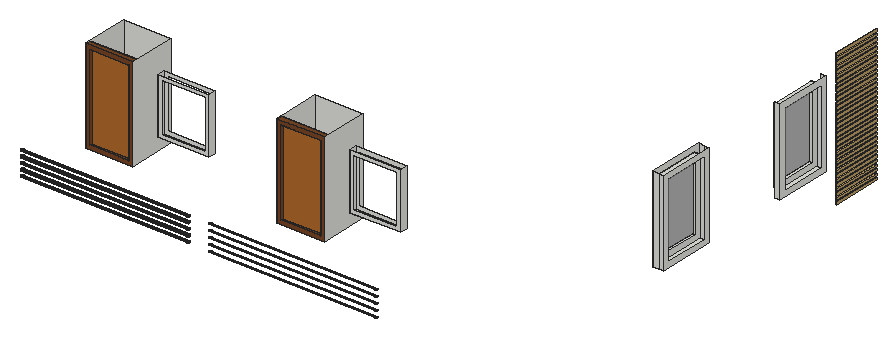
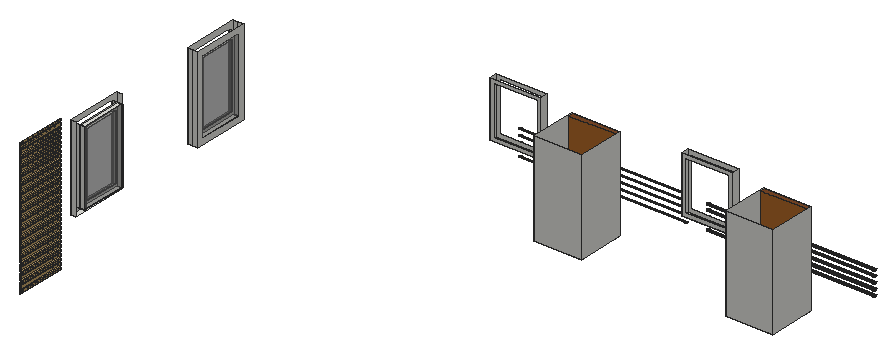
# SketchUp Ruby script. Lengths in inches.
U = 1.inch
M = Sketchup.active_model
def pt(a) = Geom::Point3d.new(a.map { |v| v * U })
def face(e, loops, mat)
  f = e.add_face(loops[0].map { |a| pt(a) })
  loops[1..].each { |l| e.add_face(l.map { |a| pt(a) }).erase! }
  f.material = f.back_material = mat if mat
  f
end
# faces: each face lists its corners as indices into pts; further lists are holes
def faces(e, pts, list, mat = nil) = list.each { |f| face(e, (f[0].is_a?(Array) ? f : [f]).map { |l| l.map { |i| pts[i] } }, mat) }
# xy, xz, yz: faces in a plane at the given z, y or x. An outline is a flat list of corners, or four numbers for a rectangle; further outlines are holes
def ring(l) = l.size == 4 ? [[l[0], l[1]], [l[2], l[1]], [l[2], l[3]], [l[0], l[3]]] : l.each_slice(2).to_a
def flat(e, list, mat, &to3) = list.each { |f| face(e, (f[0].is_a?(Array) ? f : [f]).map { |l| ring(l).map { |u, v| to3.(u, v) } }, mat) }
def xy(e, z, list, mat = nil) = flat(e, list, mat) { |x, y| [x, y, z] }
def xz(e, y, list, mat = nil) = flat(e, list, mat) { |x, z| [x, y, z] }
def yz(e, x, list, mat = nil) = flat(e, list, mat) { |y, z| [x, y, z] }
def lines(e, pts, list) = list.each { |a, b| e.add_line(pt(pts[a]), pt(pts[b])) }
# prism: a flat outline (further loops are holes) pulled along v
def prism(e, loops, v, mat = nil)
  f = face(e, loops, mat); d = Geom::Vector3d.new(v.map { |x| x * U })
  f.pushpull(f.normal.samedirection?(d) ? d.length : -d.length)
end
def box(e, o, s, mat = nil) = prism(e, [[o, [o[0] + s[0], o[1], o[2]], [o[0] + s[0], o[1] + s[1], o[2]], [o[0], o[1] + s[1], o[2]]]], [0, 0, s[2]], mat)
def at(x, y, z, deg = 0) = Geom::Transformation.translation(pt([x, y, z])) * Geom::Transformation.rotation(ORIGIN, Z_AXIS, deg.degrees)
def axes(o, x, y, z) = Geom::Transformation.new([*x, 0, *y, 0, *z, 0, *pt(o).to_a, 1])
def part(name) = M.definitions.add(name)
# library, detail: a bought-in or finely detailed component or shape, given as its bounding box
def library(name, o, s) = part(name).tap { |d| box(d.entities, o, s) }
def detail(e, o, s) = box(e.add_group.entities, o, s)
def put(e, d, t, mat = nil) = e.add_instance(d, t).tap { |i| i.material = mat if mat }
def group(e, t, mat = nil) = e.add_group.tap { |g| g.transformation = t; g.material = mat if mat }.entities
root = M.entities
M.materials.add("Generic").color = [191, 159, 103]
M.materials.add("[Translucent Glass Gray]").color = [128, 128, 128]
M.materials["[Translucent Glass Gray]"].alpha = 0.5
M.materials.add("[Wood Bamboo]").color = [177, 105, 43]
M.materials.add("[Wood Veneer 01]").color = [120, 70, 37]
c1 = part("Group\#5")
xy(c1.entities,0,[[0,0,1,57.75]])
xy(c1.entities,2.57,[[0,0,1,57.75]])
xz(c1.entities,0,[[0,0,1,2.57]])
xz(c1.entities,57.75,[[0,0,1,2.57]])
yz(c1.entities,1,[[0,0,57.75,2.57]])
c2 = part("Group\#6")
put(c2.entities,c1,at(0,0,4.75))
put(c2.entities,c1,at(0,0,0))
put(c2.entities,c1,at(0,0,19))
put(c2.entities,c1,at(0,0,28.5))
put(c2.entities,c1,at(0,0,133))
put(c2.entities,c1,at(0,0,152))
put(c2.entities,c1,at(0,0,128.25))
put(c2.entities,c1,at(0,0,9.5))
put(c2.entities,c1,at(0,0,123.5))
put(c2.entities,c1,at(0,0,114))
put(c2.entities,c1,at(0,0,147.25))
put(c2.entities,c1,at(0,0,118.75))
put(c2.entities,c1,at(0,0,142.5))
put(c2.entities,c1,at(0,0,109.25))
put(c2.entities,c1,at(0,0,137.75))
put(c2.entities,c1,at(0,0,104.5))
put(c2.entities,c1,at(0,0,99.75))
put(c2.entities,c1,at(0,0,95))
put(c2.entities,c1,at(0,0,85.5))
put(c2.entities,c1,at(0,0,80.75))
put(c2.entities,c1,at(0,0,90.25))
put(c2.entities,c1,at(0,0,76))
put(c2.entities,c1,at(0,0,71.25))
put(c2.entities,c1,at(0,0,38))
put(c2.entities,c1,at(0,0,14.25))
put(c2.entities,c1,at(0,0,33.25))
put(c2.entities,c1,at(0,0,57))
put(c2.entities,c1,at(0,0,23.75))
put(c2.entities,c1,at(0,0,61.75))
put(c2.entities,c1,at(0,0,156.75))
put(c2.entities,c1,at(0,0,47.5))
put(c2.entities,c1,at(0,0,52.25))
put(c2.entities,c1,at(0,0,42.75))
put(c2.entities,c1,at(0,0,66.5))
c3 = part("Group\#4")
xy(c3.entities,0,[[0,0,55.6875,6]],"[Wood Veneer 01]")
xy(c3.entities,4.75,[[4.75,0,50.9375,3]],"[Wood Veneer 01]")
xy(c3.entities,105.5,[[4.75,0,50.9375,3]],"[Wood Veneer 01]")
xy(c3.entities,110.25,[[0,0,55.6875,6]],"[Wood Veneer 01]")
xz(c3.entities,0,[[[0,0,55.6875,110.25],[4.75,4.75,50.9375,105.5]]],"[Wood Veneer 01]")
xz(c3.entities,3,[[4.75,4.75,50.9375,105.5]],"[Wood Bamboo]")
xz(c3.entities,6,[[0,0,55.6875,110.25]],"[Wood Bamboo]")
yz(c3.entities,0,[[0,0,6,110.25]],"[Wood Veneer 01]")
yz(c3.entities,4.75,[[0,4.75,3,105.5]],"[Wood Veneer 01]")
yz(c3.entities,50.9375,[[0,4.75,3,105.5]],"[Wood Veneer 01]")
yz(c3.entities,55.6875,[[0,0,6,110.25]],"[Wood Veneer 01]")
c4 = part("Group\#7")
xy(c4.entities,0,[[0,0,6,54.3125]])
xy(c4.entities,5.9,[[3,5.9,6,48.41]])
xy(c4.entities,81.98,[[3,5.9,6,48.41]])
xy(c4.entities,87.88,[[0,0,6,54.3125]])
xz(c4.entities,0,[[0,0,6,87.88]])
xz(c4.entities,5.9,[[3,5.9,6,81.98]])
xz(c4.entities,48.41,[[3,5.9,6,81.98]])
xz(c4.entities,54.3125,[[0,0,6,87.88]])
yz(c4.entities,0,[[0,0,54.3125,87.88]],"[Translucent Glass Gray]")
yz(c4.entities,3,[[5.9,5.9,48.41,81.98]],"[Translucent Glass Gray]")
yz(c4.entities,6,[[[0,0,54.3125,87.88],[5.9,5.9,48.41,81.98]]])
xy(root,234.72,[[214.375,158.75,270.0625,214.75],[439.6875,158.75,495.375,214.75]])
xy(root,272.84,[[802.875,257.24,809.375,324.36],[809.375,257.24,815.3125,324.36],[809.375,428.47,815.3125,495.59]])
xy(root,279.25,[[802.875,263.64,815.3125,317.96],[802.875,434.88,815.3125,489.19]])
xy(root,282.21,[[306.72,150.125,366.62,158.75],[532.04,150.125,591.93,158.75]])
xz(root,150.125,[[[306.72,282.21,366.62,348.04],[310.76,286.25,362.58,344]],[[532.04,282.21,591.93,348.04],[536.08,286.25,587.89,344]]])
xz(root,158.75,[[[306.72,282.21,366.62,348.04],[310.76,286.25,362.58,344]],[[532.04,282.21,591.93,348.04],[536.08,286.25,587.89,344]]])
xz(root,214.75,[[214.375,234.72,270.0625,344.97],[439.6875,234.72,495.375,344.97]])
xz(root,257.24,[[802.875,272.84,809.375,373.53],[809.375,272.84,815.3125,373.53]])
xz(root,263.64,[[802.875,279.25,815.3125,367.13]])
xz(root,317.96,[[802.875,279.25,815.3125,367.13]])
xz(root,324.36,[[802.875,272.84,809.375,373.53],[809.375,272.84,815.3125,373.53]])
xz(root,428.47,[[809.375,272.84,815.3125,373.53]])
xz(root,434.88,[[802.875,279.25,815.3125,367.13]])
xz(root,489.19,[[802.875,279.25,815.3125,367.13]])
xz(root,495.59,[[809.375,272.84,815.3125,373.53]])
yz(root,214.375,[[158.75,234.72,214.75,344.97]])
yz(root,270.0625,[[158.75,234.72,214.75,344.97]])
yz(root,306.72,[[150.125,282.21,158.75,348.04]])
yz(root,366.62,[[150.125,282.21,158.75,348.04]])
yz(root,439.6875,[[158.75,234.72,214.75,344.97]])
yz(root,495.375,[[158.75,234.72,214.75,344.97]])
yz(root,532.04,[[150.125,282.21,158.75,348.04]])
yz(root,591.93,[[150.125,282.21,158.75,348.04]])
yz(root,802.875,[[[257.24,272.84,324.36,373.53],[263.64,279.25,317.96,367.13]]])
yz(root,815.3125,[[[257.24,272.84,324.36,373.53],[263.64,279.25,317.96,367.13]],[[428.47,272.84,495.59,373.53],[434.88,279.25,489.19,367.13]]])
p = [[415.53,88.8125,226.625],[415.53,88.93,226.54],[613.23,88.93,226.54],[613.23,88.8125,226.625],[415.53,89.0625,226.48],[613.23,89.0625,226.48],
  [415.53,89.21,226.46],[613.23,89.21,226.46],[415.53,89.36,226.48],[613.23,89.36,226.48],[415.53,89.49,226.54],[613.23,89.49,226.54],
  [415.53,89.61,226.625],[613.23,89.61,226.625],[415.53,88.72,226.74],[613.23,88.72,226.74],[415.53,89.7,226.74],[613.23,89.7,226.74],
  [415.53,88.67,226.88],[613.23,88.67,226.88],[415.53,89.75,226.88],[613.23,89.75,226.88],[415.53,88.65,227.02],[613.23,88.65,227.02],
  [415.53,89.77,227.02],[613.23,89.77,227.02],[415.53,88.67,227.17],[613.23,88.67,227.17],[415.53,89.75,227.17],[613.23,89.75,227.17],
  [193.83,89.44,227.24],[193.83,89.73,227.125],[391.53,89.73,227.125],[391.53,89.44,227.24],[193.83,90.04,227.08],[391.53,90.04,227.08],
  [193.83,90.35,227.125],[391.53,90.35,227.125],[193.83,90.63,227.24],[391.53,90.63,227.24],[415.53,88.72,227.31],[613.23,88.72,227.31],
  [193.83,89.2,227.43],[391.53,89.2,227.43],[415.53,89.7,227.31],[613.23,89.7,227.31],[193.83,90.88,227.43],[391.53,90.88,227.43],
  [415.53,88.8125,227.42],[613.23,88.8125,227.42],[415.53,89.61,227.42],[613.23,89.61,227.42],[415.53,88.93,227.51],[613.23,88.93,227.51],
  [193.83,89.01,227.68],[391.53,89.01,227.68],[415.53,89.49,227.51],[613.23,89.49,227.51],[193.83,91.07,227.68],[391.53,91.07,227.68],
  [415.53,89.0625,227.57],[613.23,89.0625,227.57],[415.53,89.36,227.57],[613.23,89.36,227.57],[415.53,89.21,227.59],[613.23,89.21,227.59],
  [193.83,88.89,227.96],[391.53,88.89,227.96],[193.83,91.18,227.96],[391.53,91.18,227.96],[193.83,88.85,228.27],[391.53,88.85,228.27],
  [193.83,91.23,228.27],[391.53,91.23,228.27],[193.83,88.89,228.58],[391.53,88.89,228.58],[193.83,91.18,228.58],[391.53,91.18,228.58],
  [193.83,89.01,228.86],[391.53,89.01,228.86],[193.83,91.07,228.86],[391.53,91.07,228.86],[193.83,89.2,229.11],[391.53,89.2,229.11],
  [193.83,90.88,229.11],[391.53,90.88,229.11],[193.83,89.44,229.3],[391.53,89.44,229.3],[193.83,90.63,229.3],[391.53,90.63,229.3],
  [193.83,89.73,229.42],[391.53,89.73,229.42],[193.83,90.35,229.42],[391.53,90.35,229.42],[193.83,90.04,229.46],[391.53,90.04,229.46],
  [415.53,89.0625,233.86],[415.53,89.21,233.84],[613.23,89.21,233.84],[613.23,89.0625,233.86],[415.53,89.36,233.86],[613.23,89.36,233.86],
  [193.83,89.44,233.93],[193.83,89.73,233.8125],[391.53,89.73,233.8125],[391.53,89.44,233.93],[193.83,90.04,233.77],[391.53,90.04,233.77],
  [193.83,90.35,233.8125],[391.53,90.35,233.8125],[193.83,90.63,233.93],[391.53,90.63,233.93],[415.53,88.8125,234],[415.53,88.93,233.91],
  [613.23,88.93,233.91],[613.23,88.8125,234],[193.83,89.2,234.12],[391.53,89.2,234.12],[415.53,89.49,233.91],[613.23,89.49,233.91],
  [415.53,89.61,234],[613.23,89.61,234],[193.83,90.88,234.12],[391.53,90.88,234.12],[415.53,88.72,234.12],[613.23,88.72,234.12],
  [415.53,89.7,234.12],[613.23,89.7,234.12],[415.53,88.67,234.25],[613.23,88.67,234.25],[193.83,89.01,234.36],[391.53,89.01,234.36],
  [415.53,89.75,234.25],[613.23,89.75,234.25],[193.83,91.07,234.36],[391.53,91.07,234.36],[415.53,88.65,234.4],[613.23,88.65,234.4],
  [415.53,89.77,234.4],[613.23,89.77,234.4],[415.53,88.67,234.54],[613.23,88.67,234.54],[193.83,88.89,234.65],[391.53,88.89,234.65],
  [415.53,89.75,234.54],[613.23,89.75,234.54],[193.83,91.18,234.65],[391.53,91.18,234.65],[415.53,88.72,234.68],[613.23,88.72,234.68],
  [415.53,89.7,234.68],[613.23,89.7,234.68],[415.53,88.8125,234.8],[613.23,88.8125,234.8],[193.83,88.85,234.96],[391.53,88.85,234.96],
  [415.53,89.61,234.8],[613.23,89.61,234.8],[193.83,91.23,234.96],[391.53,91.23,234.96],[415.53,88.93,234.89],[613.23,88.93,234.89],
  [415.53,89.49,234.89],[613.23,89.49,234.89],[415.53,89.0625,234.94],[613.23,89.0625,234.94],[415.53,89.21,234.96],[613.23,89.21,234.96],
  [415.53,89.36,234.94],[613.23,89.36,234.94],[193.83,88.89,235.27],[391.53,88.89,235.27],[193.83,91.18,235.27],[391.53,91.18,235.27],
  [193.83,89.01,235.55],[391.53,89.01,235.55],[193.83,91.07,235.55],[391.53,91.07,235.55],[193.83,89.2,235.8],[391.53,89.2,235.8],
  [193.83,90.88,235.8],[391.53,90.88,235.8],[193.83,89.44,235.99],[391.53,89.44,235.99],[193.83,90.63,235.99],[391.53,90.63,235.99],
  [193.83,89.73,236.11],[391.53,89.73,236.11],[193.83,90.35,236.11],[391.53,90.35,236.11],[193.83,90.04,236.15],[391.53,90.04,236.15],
  [193.83,89.44,240.93],[193.83,89.73,240.8125],[391.53,89.73,240.8125],[391.53,89.44,240.93],[193.83,90.04,240.77],[391.53,90.04,240.77],
  [193.83,90.35,240.8125],[391.53,90.35,240.8125],[193.83,90.63,240.93],[391.53,90.63,240.93],[193.83,89.2,241.12],[391.53,89.2,241.12],
  [193.83,90.88,241.12],[391.53,90.88,241.12],[193.83,89.01,241.36],[391.53,89.01,241.36],[193.83,91.07,241.36],[391.53,91.07,241.36],
  [415.53,89.0625,241.36],[415.53,89.21,241.34],[613.23,89.21,241.34],[613.23,89.0625,241.36],[415.53,89.36,241.36],[613.23,89.36,241.36],
  [415.53,88.8125,241.5],[415.53,88.93,241.41],[613.23,88.93,241.41],[613.23,88.8125,241.5],[193.83,88.89,241.65],[391.53,88.89,241.65],
  [415.53,89.49,241.41],[613.23,89.49,241.41],[415.53,89.61,241.5],[613.23,89.61,241.5],[193.83,91.18,241.65],[391.53,91.18,241.65],
  [415.53,88.72,241.62],[613.23,88.72,241.62],[415.53,89.7,241.62],[613.23,89.7,241.62],[415.53,88.67,241.75],[613.23,88.67,241.75],
  [415.53,89.75,241.75],[613.23,89.75,241.75],[193.83,88.85,241.96],[391.53,88.85,241.96],[193.83,91.23,241.96],[391.53,91.23,241.96],
  [415.53,88.65,241.9],[613.23,88.65,241.9],[415.53,89.77,241.9],[613.23,89.77,241.9],[415.53,88.67,242.04],[613.23,88.67,242.04],
  [415.53,89.75,242.04],[613.23,89.75,242.04],[415.53,88.72,242.18],[613.23,88.72,242.18],[193.83,88.89,242.27],[391.53,88.89,242.27],
  [415.53,89.7,242.18],[613.23,89.7,242.18],[193.83,91.18,242.27],[391.53,91.18,242.27],[415.53,88.8125,242.3],[613.23,88.8125,242.3],
  [415.53,89.61,242.3],[613.23,89.61,242.3],[415.53,88.93,242.39],[613.23,88.93,242.39],[193.83,89.01,242.55],[391.53,89.01,242.55],
  [415.53,89.49,242.39],[613.23,89.49,242.39],[193.83,91.07,242.55],[391.53,91.07,242.55],[415.53,89.0625,242.44],[613.23,89.0625,242.44],
  [415.53,89.21,242.46],[613.23,89.21,242.46],[415.53,89.36,242.44],[613.23,89.36,242.44],[193.83,89.2,242.8],[391.53,89.2,242.8],
  [193.83,90.88,242.8],[391.53,90.88,242.8],[193.83,89.44,242.99],[391.53,89.44,242.99],[193.83,90.63,242.99],[391.53,90.63,242.99],
  [193.83,89.73,243.11],[391.53,89.73,243.11],[193.83,90.35,243.11],[391.53,90.35,243.11],[193.83,90.04,243.15],[391.53,90.04,243.15],
  [193.83,89.44,247.93],[193.83,89.73,247.8125],[391.53,89.73,247.8125],[391.53,89.44,247.93],[193.83,90.04,247.77],[391.53,90.04,247.77],
  [193.83,90.35,247.8125],[391.53,90.35,247.8125],[193.83,90.63,247.93],[391.53,90.63,247.93],[193.83,89.2,248.12],[391.53,89.2,248.12],
  [193.83,90.88,248.12],[391.53,90.88,248.12],[193.83,89.01,248.36],[391.53,89.01,248.36],[193.83,91.07,248.36],[391.53,91.07,248.36],
  [193.83,88.89,248.65],[391.53,88.89,248.65],[193.83,91.18,248.65],[391.53,91.18,248.65],[193.83,88.85,248.96],[391.53,88.85,248.96],
  [193.83,91.23,248.96],[391.53,91.23,248.96],[415.53,89.0625,248.86],[415.53,89.21,248.84],[613.23,89.21,248.84],[613.23,89.0625,248.86],
  [415.53,89.36,248.86],[613.23,89.36,248.86],[415.53,88.8125,249],[415.53,88.93,248.91],[613.23,88.93,248.91],[613.23,88.8125,249],
  [415.53,89.49,248.91],[613.23,89.49,248.91],[415.53,89.61,249],[613.23,89.61,249],[415.53,88.72,249.12],[613.23,88.72,249.12],
  [193.83,88.89,249.27],[391.53,88.89,249.27],[415.53,89.7,249.12],[613.23,89.7,249.12],[193.83,91.18,249.27],[391.53,91.18,249.27],
  [415.53,88.67,249.25],[613.23,88.67,249.25],[415.53,89.75,249.25],[613.23,89.75,249.25],[415.53,88.65,249.4],[613.23,88.65,249.4],
  [193.83,89.01,249.55],[391.53,89.01,249.55],[415.53,89.77,249.4],[613.23,89.77,249.4],[193.83,91.07,249.55],[391.53,91.07,249.55],
  [415.53,88.67,249.54],[613.23,88.67,249.54],[415.53,89.75,249.54],[613.23,89.75,249.54],[415.53,88.72,249.68],[613.23,88.72,249.68],
  [415.53,89.7,249.68],[613.23,89.7,249.68],[193.83,89.2,249.8],[391.53,89.2,249.8],[193.83,90.88,249.8],[391.53,90.88,249.8],
  [415.53,88.8125,249.8],[613.23,88.8125,249.8],[415.53,89.61,249.8],[613.23,89.61,249.8],[415.53,88.93,249.89],[613.23,88.93,249.89],
  [193.83,89.44,249.99],[391.53,89.44,249.99],[415.53,89.49,249.89],[613.23,89.49,249.89],[193.83,90.63,249.99],[391.53,90.63,249.99],
  [415.53,89.0625,249.94],[613.23,89.0625,249.94],[415.53,89.21,249.96],[613.23,89.21,249.96],[415.53,89.36,249.94],[613.23,89.36,249.94],
  [193.83,89.73,250.11],[391.53,89.73,250.11],[193.83,90.35,250.11],[391.53,90.35,250.11],[193.83,90.04,250.15],[391.53,90.04,250.15],
  [193.83,89.73,254.375],[193.83,90.04,254.33],[391.53,90.04,254.33],[391.53,89.73,254.375],[193.83,90.35,254.375],[391.53,90.35,254.375],
  [193.83,89.44,254.49],[391.53,89.44,254.49],[193.83,90.63,254.49],[391.53,90.63,254.49],[193.83,89.2,254.68],[391.53,89.2,254.68],
  [193.83,90.88,254.68],[391.53,90.88,254.68],[193.83,89.01,254.93],[391.53,89.01,254.93],[193.83,91.07,254.93],[391.53,91.07,254.93],
  [193.83,88.89,255.21],[391.53,88.89,255.21],[193.83,91.18,255.21],[391.53,91.18,255.21],[193.83,88.85,255.52],[391.53,88.85,255.52],
  [193.83,91.23,255.52],[391.53,91.23,255.52],[193.83,88.89,255.83],[391.53,88.89,255.83],[193.83,91.18,255.83],[391.53,91.18,255.83],
  [193.83,89.01,256.11],[391.53,89.01,256.11],[193.83,91.07,256.11],[391.53,91.07,256.11],[193.83,89.2,256.36],[391.53,89.2,256.36],
  [193.83,90.88,256.36],[391.53,90.88,256.36],[415.53,88.8125,256.4375],[415.53,88.93,256.35],[613.23,88.93,256.35],[613.23,88.8125,256.4375],
  [415.53,89.0625,256.29],[613.23,89.0625,256.29],[415.53,89.21,256.27],[613.23,89.21,256.27],[415.53,89.36,256.29],[613.23,89.36,256.29],
  [415.53,89.49,256.35],[613.23,89.49,256.35],[415.53,89.61,256.4375],[613.23,89.61,256.4375],[415.53,88.72,256.56],[613.23,88.72,256.56],
  [193.83,89.44,256.55],[391.53,89.44,256.55],[415.53,89.7,256.56],[613.23,89.7,256.56],[193.83,90.63,256.55],[391.53,90.63,256.55],
  [193.83,89.73,256.67],[391.53,89.73,256.67],[193.83,90.35,256.67],[391.53,90.35,256.67],[415.53,88.67,256.69],[613.23,88.67,256.69],
  [415.53,89.75,256.69],[613.23,89.75,256.69],[415.53,88.65,256.84],[613.23,88.65,256.84],[193.83,90.04,256.71],[391.53,90.04,256.71],
  [415.53,89.77,256.84],[613.23,89.77,256.84],[415.53,88.67,256.98],[613.23,88.67,256.98],[415.53,89.75,256.98],[613.23,89.75,256.98],
  [415.53,88.72,257.12],[613.23,88.72,257.12],[415.53,89.7,257.12],[613.23,89.7,257.12],[415.53,88.8125,257.23],[613.23,88.8125,257.23],
  [415.53,89.61,257.23],[613.23,89.61,257.23],[415.53,88.93,257.32],[613.23,88.93,257.32],[415.53,89.49,257.32],[613.23,89.49,257.32],
  [415.53,89.0625,257.38],[613.23,89.0625,257.38],[415.53,89.36,257.38],[613.23,89.36,257.38],[415.53,89.21,257.4],[613.23,89.21,257.4],
  [415.53,89.21,227.02],[613.23,89.21,227.02],[415.53,89.21,234.46],[613.23,89.21,234.46],[415.53,89.21,241.9],[613.23,89.21,241.9],
  [415.53,89.21,249.34],[613.23,89.21,249.34],[415.53,89.21,256.77],[613.23,89.21,256.77],[193.83,90.04,228.65],[391.53,90.04,228.65],
  [193.83,90.04,235.4],[391.53,90.04,235.4],[193.83,90.04,242.15],[391.53,90.04,242.15],[193.83,90.04,248.9],[391.53,90.04,248.9],
  [193.83,90.04,255.65],[391.53,90.04,255.65]]
faces(root,p,[[0,1,2,3],[1,4,5,2],[4,6,7,5],[6,8,9,7],[8,10,11,9],[10,12,13,11],[14,0,3,15],[12,16,17,13],
  [18,14,15,19],[16,20,21,17],[22,18,19,23],[20,24,25,21],[26,22,23,27],[24,28,29,25],[30,31,32,33],[31,34,35,32],
  [34,36,37,35],[36,38,39,37],[40,26,27,41],[42,30,33,43],[28,44,45,29],[38,46,47,39],[48,40,41,49],[44,50,51,45],
  [52,48,49,53],[54,42,43,55],[50,56,57,51],[46,58,59,47],[60,52,53,61],[56,62,63,57],[64,60,61,65],[62,64,65,63],
  [66,54,55,67],[58,68,69,59],[70,66,67,71],[68,72,73,69],[74,70,71,75],[72,76,77,73],[78,74,75,79],[76,80,81,77],
  [82,78,79,83],[80,84,85,81],[86,82,83,87],[84,88,89,85],[90,86,87,91],[88,92,93,89],[94,90,91,95],[92,94,95,93],
  [96,97,98,99],[97,100,101,98],[102,103,104,105],[103,106,107,104],[106,108,109,107],[108,110,111,109],[112,113,114,115],[113,96,99,114],
  [116,102,105,117],[100,118,119,101],[118,120,121,119],[110,122,123,111],[124,112,115,125],[120,126,127,121],[128,124,125,129],[130,116,117,131],
  [126,132,133,127],[122,134,135,123],[136,128,129,137],[132,138,139,133],[140,136,137,141],[142,130,131,143],[138,144,145,139],[134,146,147,135],
  [148,140,141,149],[144,150,151,145],[152,148,149,153],[154,142,143,155],[150,156,157,151],[146,158,159,147],[160,152,153,161],[156,162,163,157],
  [164,160,161,165],[166,164,165,167],[168,166,167,169],[162,168,169,163],[170,154,155,171],[158,172,173,159],[174,170,171,175],[172,176,177,173],
  [178,174,175,179],[176,180,181,177],[182,178,179,183],[180,184,185,181],[186,182,183,187],[184,188,189,185],[190,186,187,191],[188,190,191,189],
  [192,193,194,195],[193,196,197,194],[196,198,199,197],[198,200,201,199],[202,192,195,203],[200,204,205,201],[206,202,203,207],[204,208,209,205],
  [210,211,212,213],[211,214,215,212],[216,217,218,219],[220,206,207,221],[217,210,213,218],[214,222,223,215],[222,224,225,223],[208,226,227,209],
  [228,216,219,229],[224,230,231,225],[232,228,229,233],[230,234,235,231],[236,220,221,237],[226,238,239,227],[240,232,233,241],[234,242,243,235],
  [244,240,241,245],[242,246,247,243],[248,244,245,249],[250,236,237,251],[246,252,253,247],[238,254,255,239],[256,248,249,257],[252,258,259,253],
  [260,256,257,261],[262,250,251,263],[258,264,265,259],[254,266,267,255],[268,260,261,269],[270,268,269,271],[272,270,271,273],[264,272,273,265],
  [274,262,263,275],[266,276,277,267],[278,274,275,279],[276,280,281,277],[282,278,279,283],[280,284,285,281],[286,282,283,287],[284,286,287,285],
  [288,289,290,291],[289,292,293,290],[292,294,295,293],[294,296,297,295],[298,288,291,299],[296,300,301,297],[302,298,299,303],[300,304,305,301],
  [306,302,303,307],[304,308,309,305],[310,306,307,311],[308,312,313,309],[314,315,316,317],[315,318,319,316],[320,321,322,323],[321,314,317,322],
  [318,324,325,319],[324,326,327,325],[328,320,323,329],[330,310,311,331],[326,332,333,327],[312,334,335,313],[336,328,329,337],[332,338,339,333],
  [340,336,337,341],[342,330,331,343],[338,344,345,339],[334,346,347,335],[348,340,341,349],[344,350,351,345],[352,348,349,353],[350,354,355,351],
  [356,342,343,357],[346,358,359,347],[360,352,353,361],[354,362,363,355],[364,360,361,365],[366,356,357,367],[362,368,369,363],[358,370,371,359],
  [372,364,365,373],[374,372,373,375],[376,374,375,377],[368,376,377,369],[378,366,367,379],[370,380,381,371],[382,378,379,383],[380,382,383,381],
  [384,385,386,387],[385,388,389,386],[390,384,387,391],[388,392,393,389],[394,390,391,395],[392,396,397,393],[398,394,395,399],[396,400,401,397],
  [402,398,399,403],[400,404,405,401],[406,402,403,407],[404,408,409,405],[410,406,407,411],[408,412,413,409],[414,410,411,415],[412,416,417,413],
  [418,414,415,419],[416,420,421,417],[422,423,424,425],[423,426,427,424],[426,428,429,427],[428,430,431,429],[430,432,433,431],[432,434,435,433],
  [436,422,425,437],[438,418,419,439],[434,440,441,435],[420,442,443,421],[444,438,439,445],[442,446,447,443],[448,436,437,449],[440,450,451,441],
  [452,448,449,453],[454,444,445,455],[450,456,457,451],[446,454,455,447],[458,452,453,459],[456,460,461,457],[462,458,459,463],[460,464,465,461],
  [466,462,463,467],[464,468,469,465],[470,466,467,471],[468,472,473,469],[474,470,471,475],[472,476,477,473],[478,474,475,479],[476,478,479,477]])
lines(root,p,[[480,481],[482,483],[484,485],[486,487],[488,489],[490,491],[492,493],[494,495],[496,497],[498,499]])
put(root,c2,at(809.4375,518.09,226.8125),"Generic")
put(root,c3,at(439.6875,158.75,234.72))
put(root,c3,at(214.375,158.75,234.72))
put(root,c4,at(803.375,434.88,279.25))
put(root,c4,at(803.375,263.64,279.25))
